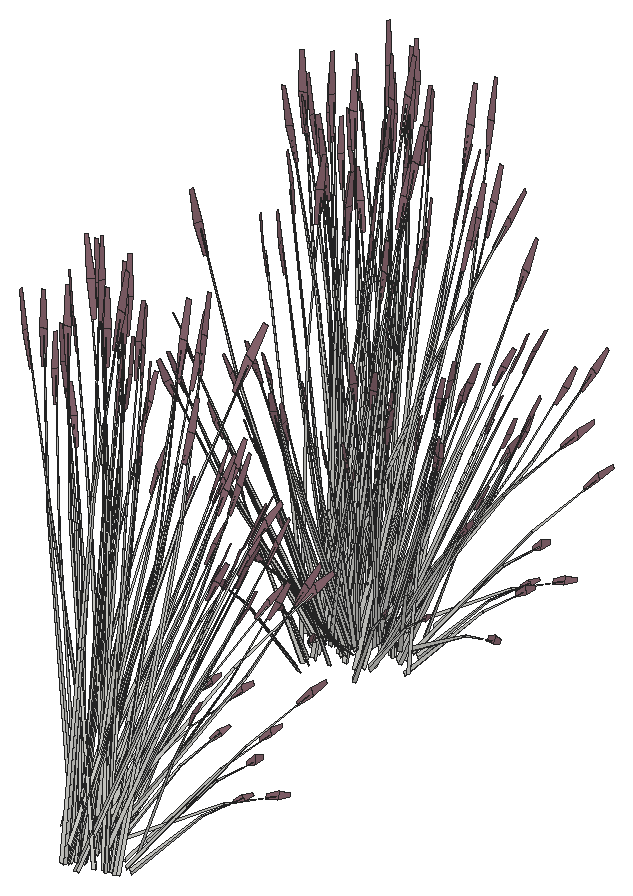
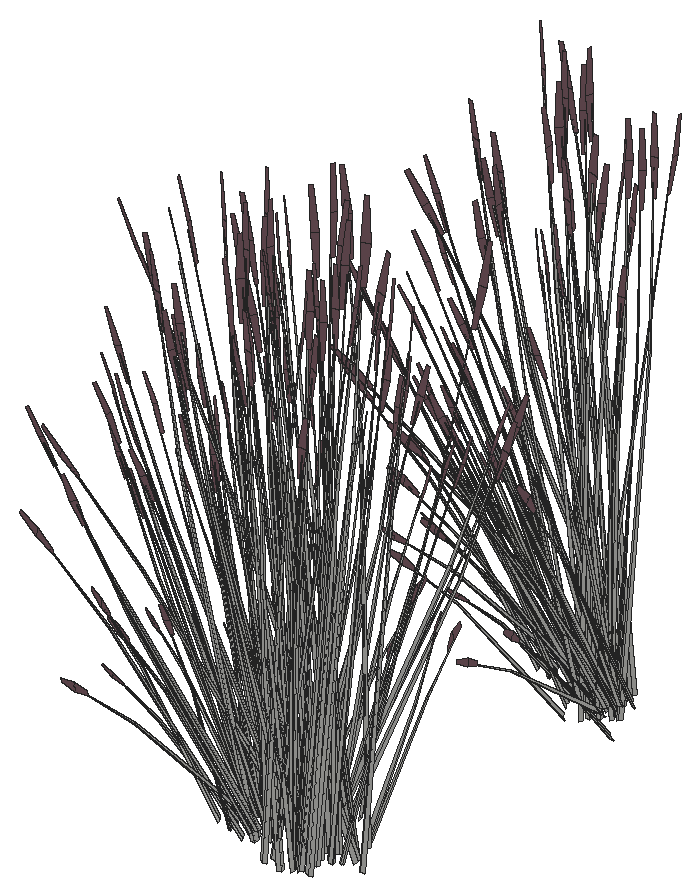
# SketchUp Ruby script. Lengths in inches.
U = 1.inch
M = Sketchup.active_model
def pt(a) = Geom::Point3d.new(a.map { |v| v * U })
def face(e, loops, mat)
  f = e.add_face(loops[0].map { |a| pt(a) })
  loops[1..].each { |l| e.add_face(l.map { |a| pt(a) }).erase! }
  f.material = f.back_material = mat if mat
  f
end
# faces: each face lists its corners as indices into pts; further lists are holes
def faces(e, pts, list, mat = nil) = list.each { |f| face(e, (f[0].is_a?(Array) ? f : [f]).map { |l| l.map { |i| pts[i] } }, mat) }
# xy, xz, yz: faces in a plane at the given z, y or x. An outline is a flat list of corners, or four numbers for a rectangle; further outlines are holes
def ring(l) = l.size == 4 ? [[l[0], l[1]], [l[2], l[1]], [l[2], l[3]], [l[0], l[3]]] : l.each_slice(2).to_a
def flat(e, list, mat, &to3) = list.each { |f| face(e, (f[0].is_a?(Array) ? f : [f]).map { |l| ring(l).map { |u, v| to3.(u, v) } }, mat) }
def xy(e, z, list, mat = nil) = flat(e, list, mat) { |x, y| [x, y, z] }
def xz(e, y, list, mat = nil) = flat(e, list, mat) { |x, z| [x, y, z] }
def yz(e, x, list, mat = nil) = flat(e, list, mat) { |y, z| [x, y, z] }
def lines(e, pts, list) = list.each { |a, b| e.add_line(pt(pts[a]), pt(pts[b])) }
# prism: a flat outline (further loops are holes) pulled along v
def prism(e, loops, v, mat = nil)
  f = face(e, loops, mat); d = Geom::Vector3d.new(v.map { |x| x * U })
  f.pushpull(f.normal.samedirection?(d) ? d.length : -d.length)
end
def box(e, o, s, mat = nil) = prism(e, [[o, [o[0] + s[0], o[1], o[2]], [o[0] + s[0], o[1] + s[1], o[2]], [o[0], o[1] + s[1], o[2]]]], [0, 0, s[2]], mat)
def at(x, y, z, deg = 0) = Geom::Transformation.translation(pt([x, y, z])) * Geom::Transformation.rotation(ORIGIN, Z_AXIS, deg.degrees)
def axes(o, x, y, z) = Geom::Transformation.new([*x, 0, *y, 0, *z, 0, *pt(o).to_a, 1])
def part(name) = M.definitions.add(name)
# library, detail: a bought-in or finely detailed component or shape, given as its bounding box
def library(name, o, s) = part(name).tap { |d| box(d.entities, o, s) }
def detail(e, o, s) = box(e.add_group.entities, o, s)
def put(e, d, t, mat = nil) = e.add_instance(d, t).tap { |i| i.material = mat if mat }
def group(e, t, mat = nil) = e.add_group.tap { |g| g.transformation = t; g.material = mat if mat }.entities
root = M.entities
M.materials.add("LightPink_Translucent").color = [144, 107, 117]
c1 = part("blade")
p = [[2.15,0.21,22],[0,0.17,0],[0.09,0.45,0],[2.18,0.31,22],[2.29,0.31,22],[0.38,0.45,0],
  [2.48,0.24,33],[2.49,0.24,33],[2.48,0.22,33]]
faces(c1.entities,p,[[0,1,2,3],[4,5,2,3],[6,3,4,7],[8,0,3,6]])
c2 = part("seeds")
p = [[0.3,-0.1,1.38],[-0.01,-0.03,1.59],[-0.01,-0.03,0.03],[0.14,-0.07,-0.07],[0.29,-0.03,3],[0.15,0.01,3.11]]
faces(c2.entities,p,[[0,1,2,3],[1,0,4,5]],"LightPink_Translucent")
c3 = part("blade with seeds")
put(c3.entities,c1,at(0,0,0))
put(c3.entities,c2,axes([2.4,0.25,30.99],[1.5799,-0.05474,1.17369],[-0.12525,1.92788,0.29478],[-0.07173,-0.02425,1.56792]))
put(root,c3,axes([73.33,431.42,34.53],[-0.50328,-1.06202,-0.69835],[1.44974,-0.38248,-0.18329],[-0.05563,-0.35963,1.54149]))
put(root,c3,axes([76.63,428.04,37.46],[-1.19922,0.48218,-0.1216],[-0.58932,-0.85579,-0.67495],[-0.15822,-0.36063,1.02557]))
put(root,c3,axes([75.6,428.08,37.11],[-1.20468,-0.25962,-0.51099],[0.41292,-0.89013,-0.3958],[-0.11046,-0.35838,0.97773]))
put(root,c3,axes([73.38,392.2,32.11],[-0.02999,-0.3975,1.71376],[1.30002,0.26369,0.13857],[-0.08041,0.56647,0.73262]))
put(root,c3,axes([70.95,431.29,34.46],[0.85545,-0.64616,-0.30978],[0.85545,0.64616,0.30978],[0,-0.20813,1.38974]))
put(root,c3,axes([74.82,427.11,34.56],[-0.84686,0.59414,-0.03893],[-0.77596,-0.65071,-0.17649],[-0.05463,-0.18438,0.58215]))
put(root,c3,axes([74.48,432.97,34.79],[1.54892,0.2182,0.45755],[-0.31522,1.23236,0.17955],[-0.22636,-0.119,1.58856]))
put(root,c3,axes([74.08,432.75,35.15],[-0.59459,0.93321,0.44739],[-1.23546,-0.44912,-0.21531],[0,-0.21512,1.43643]))
put(root,c3,axes([76.04,428.25,37.41],[-0.5849,-0.8421,-0.71045],[1.20401,-0.4693,0.08574],[-0.13677,-0.40688,1.00501]))
put(root,c3,axes([73.65,434.94,34.9],[1.31687,-0.27488,0.17642],[0.32517,1.02297,0.35086],[-0.11745,-0.14905,1.60407]))
put(root,c3,axes([75.34,392.62,30.43],[-1.23546,-0.46496,0],[0.59459,-0.96613,0],[0,0,1.62707]))
put(root,c3,axes([75.34,435.1,34.625],[-1.23546,-0.46496,0],[0.59459,-0.96613,0],[0,0,1.62707]))
put(root,c3,axes([76.27,428.375,37.48],[-0.36946,0.79643,0.35414],[-1.07787,-0.23229,-0.4572],[-0.09883,-0.32066,0.87481]))
put(root,c3,axes([78.2,393.78,30.61],[0.7662,1.03778,0],[-1.28187,0.57875,-0.51607],[-0.29196,0.13181,1.63711]))
put(root,c3,axes([74.3,394.23,33.3],[-1.20755,-0.27075,0.53283],[0.41292,-0.89013,0.43934],[0.07257,0.35005,1.10256]))
put(root,c3,axes([73.98,394.3,32.97],[-0.90301,0.35198,0.0643],[-0.44199,-0.64184,0.50621],[0.08721,0.28293,0.77189]))
put(root,c3,axes([77.5625,392.51,30.71],[0.35402,-1.02926,0.17642],[1.29548,0.29127,0.35086],[-0.22379,0.00501,1.60407]))
put(root,c3,axes([77.5625,435,34.9],[0.35402,-1.02926,0.17642],[1.29548,0.29127,0.35086],[-0.22379,0.00501,1.60407]))
put(root,c3,axes([76.97,391.15,30.85],[0.90538,0.62224,0.1448],[-0.75521,0.70202,-0.41347],[-0.21021,0.09491,1.26744]))
put(root,c3,axes([76.97,433.63,35.04],[0.90538,0.62224,0.1448],[-0.75521,0.70202,-0.41347],[-0.21021,0.09491,1.26744]))
put(root,c3,axes([76.64,432.86,34.73],[-1.1399,-0.8914,-0.06131],[1.1406,-0.89194,0],[-0.03981,-0.03113,1.75571]))
put(root,c3,axes([76.94,390.6875,30.95],[1.33077,-0.06393,0.44739],[0.12035,1.06125,-0.21531],[-0.23824,0.10756,1.43643]))
put(root,c3,axes([76.94,433.17,35.15],[1.33077,-0.06393,0.44739],[0.12035,1.06125,-0.21531],[-0.23824,0.10756,1.43643]))
put(root,c3,axes([77.27,393.13,30.57],[1.53422,0.33662,0.30756],[-0.38383,1.20322,-0.36492],[-0.25393,0.15059,1.64885]))
put(root,c3,axes([75.03,426.38,33.92],[-0.20555,0.03731,1.76342],[-1.13672,-0.42002,-0.26939],[0.01907,-0.35034,0.30037]))
put(root,c3,axes([77.93,393.0625,30.71],[1.14694,-0.51783,0.49651],[0.68554,0.92854,0],[-0.26122,0.11794,1.57504]))
put(root,c3,axes([77.93,435.55,34.91],[1.14694,-0.51783,0.49651],[0.68554,0.92854,0],[-0.26122,0.11794,1.57504]))
put(root,c3,axes([76.15,427.54,36.95],[0.36946,-0.79643,-0.35414],[1.07787,0.23229,0.4572],[-0.09883,-0.32066,0.87481]))
put(root,c3,axes([74.34,431.84,34.79],[0.53281,1.15808,0.45755],[-1.52239,0.4027,0.17955],[0.01861,-0.2128,1.58856]))
put(root,c3,axes([74.1,431.6875,34.64],[0.59459,-0.93321,-0.44739],[1.23546,0.44912,0.21531],[0,-0.21512,1.43643]))
put(root,c3,axes([75.62,392.21,30.44],[-0.39985,-0.89288,0],[1.1418,-0.31268,0],[0,0,1.54371]))
put(root,c3,axes([75.62,434.7,34.63],[-0.39985,-0.89288,0],[1.1418,-0.31268,0],[0,0,1.54371]))
put(root,c3,axes([74.17,394.1,29.73],[0.19833,-0.05635,1.76342],[1.19302,0.31018,-0.26939],[0.03489,0.3496,0.30037]))
put(root,c3,axes([74.43,394.41,32.76],[-0.36946,0.79643,-0.35414],[-1.07787,-0.23229,0.4572],[0.09883,0.32066,0.87481]))
put(root,c3,axes([77.24,390.45,30.45],[-0.59459,0.93321,-0.44739],[-1.23546,-0.44912,0.21531],[0,0.21512,1.43643]))
put(root,c3,axes([76.6,427.65,37.16],[0.90301,-0.35198,0.0643],[0.44199,0.64184,0.50621],[-0.08721,-0.28293,0.77189]))
put(root,c3,axes([73.67,395.82,32.95],[0.15534,0.16677,1.74944],[1.25362,0.06552,-0.27667],[0.12606,0.3678,0.14031]))
put(root,c3,axes([79.59,389.89,30.71],[-0.96285,-0.75439,0.17642],[0.97031,-0.7317,0.35086],[-0.10634,0.15406,1.60407]))
put(root,c3,axes([79.59,432.37,34.9],[-0.96285,-0.75439,0.17642],[0.97031,-0.7317,0.35086],[-0.10634,0.15406,1.60407]))
put(root,c3,axes([76.26,431.93,34.63],[0,-1.19833,0],[1.53239,0,0],[0,0,1.79456]))
put(root,c3,axes([76.28,427.72,37.16],[1.20755,0.27075,0.48003],[-0.41292,0.89013,0.3958],[-0.07257,-0.35005,0.9933]))
put(root,c3,axes([74.84,432.15,34.86],[1.3808,0.50196,0.24065],[-0.66454,1.04299,0.50002],[0,-0.24043,1.60543]))
put(root,c3,axes([77.03,389.93,30.53],[0,1.19774,-0.05637],[-1.53239,0,0],[0,0.03764,1.79368]))
put(root,c3,axes([77.03,432.41,34.72],[0,1.19774,-0.05637],[-1.53239,0,0],[0,0.03764,1.79368]))
put(root,c3,axes([74.39,431.45,35.15],[-1.33077,0.06393,0.44739],[-0.12035,-1.06125,-0.21531],[0.23824,-0.10756,1.43643]))
put(root,c3,axes([74.3125,393.57,33.29],[0.36946,-0.79643,0.35414],[1.07787,0.23229,-0.4572],[0.09883,0.32066,0.87481]))
put(root,c3,axes([73.77,429.63,34.9],[-0.35402,1.02926,0.17642],[-1.29548,-0.29127,0.35086],[0.22379,-0.00501,1.60407]))
put(root,c3,axes([76.3,392.25,30.53],[0.53281,1.18979,-0.06012],[-1.52239,0.41691,0],[0.01861,0.04155,1.72173]))
put(root,c3,axes([76.3,434.73,34.72],[0.53281,1.18979,-0.06012],[-1.52239,0.41691,0],[0.01861,0.04155,1.72173]))
put(root,c3,axes([73.14,428.36,34.8],[-0.7662,-1.03778,0],[1.28187,-0.57875,-0.51607],[0.29196,-0.13181,1.63711]))
put(root,c3,axes([74.54,393.7,33.22],[0.5849,0.8421,-0.71045],[-1.20401,0.4693,0.08574],[0.13677,0.40688,1.00501]))
put(root,c3,axes([80.7,390.69,30.4375],[-1.53164,-0.00828,-0.04976],[0,-1.1575,0.49943],[-0.04813,0.2635,1.58352]))
put(root,c3,axes([80.7,433.17,34.63],[-1.53164,-0.00828,-0.04976],[0,-1.1575,0.49943],[-0.04813,0.2635,1.58352]))
put(root,c3,axes([77.6875,429.6875,34.9],[-1.31687,0.27488,0.17642],[-0.32517,-1.02297,0.35086],[0.11745,0.14905,1.60407]))
put(root,c3,axes([76.34,425.85,35.19],[0.15721,0.60392,1.1486],[-0.87211,-0.33448,0.84392],[0.09385,-0.30923,0.25299]))
put(root,c3,axes([75.76,396.42,33.88],[0.84686,-0.59414,-0.06488],[0.77596,0.65071,-0.29416],[0.05463,0.18438,0.97024]))
put(root,c3,axes([75.53,431.18,34.79],[-1.01611,0.93987,0.45755],[-1.20717,-0.82966,0.17955],[0.24496,-0.0938,1.58856]))
put(root,c3,axes([77.27,390.18,30.45],[0.85545,0.66896,0],[-0.85545,0.66896,0],[0,0,1.69266]))
put(root,c3,axes([77.27,432.66,34.64],[0.85545,0.66896,0],[-0.85545,0.66896,0],[0,0,1.69266]))
put(root,c3,axes([77.26,389.39,30.95],[0.59459,-0.93321,0.44739],[1.23546,0.44912,-0.21531],[0,0.21512,1.43643]))
put(root,c3,axes([77.26,431.88,35.15],[0.59459,-0.93321,0.44739],[1.23546,0.44912,-0.21531],[0,0.21512,1.43643]))
put(root,c3,axes([76.74,392.64,30.44],[1.23546,0.46496,0],[-0.59459,0.96613,0],[0,0,1.74954]))
put(root,c3,axes([76.74,435.12,34.63],[1.23546,0.46496,0],[-0.59459,0.96613,0],[0,0,1.74954]))
put(root,c3,axes([74.98,393.87,32.92],[1.20468,0.25962,-0.51099],[-0.41292,0.89013,-0.3958],[0.11046,0.35838,0.97773]))
put(root,c3,axes([73.95,393.91,33.27],[1.19922,-0.48218,-0.1216],[0.58932,0.85579,-0.67495],[0.15822,0.36063,1.02557]))
put(root,c3,axes([76.86,389.17,30.62],[-1.54892,-0.2182,0.49198],[0.31522,-1.23236,0.19306],[0.22636,0.119,1.70813]))
put(root,c3,axes([76.86,431.66,34.81],[-1.54892,-0.2182,0.49198],[0.31522,-1.23236,0.19306],[0.22636,0.119,1.70813]))
put(root,c3,axes([80.08,426.84,37.14],[-0.12446,0.07911,1.77383],[-1.21937,-0.26689,-0.16761],[-0.04414,-0.34521,0.31391]))
put(root,c3,axes([79.12,429.125,37.46],[-1.34686,-0.05131,-0.1216],[0.03681,-0.97156,-0.67495],[0.09356,-0.37418,1.02557]))
put(root,c3,axes([80.38,390.85,30.26],[-0.85545,0.64616,-0.30978],[-0.85545,-0.64616,0.30978],[0,0.20813,1.38974]))
put(root,c3,axes([77.94,390.73,30.33],[0.44936,0.94823,-0.69212],[-1.29441,0.3415,-0.18165],[0.04967,0.32109,1.52773]))
put(root,c3,axes([77.3,432.2,34.63],[1.37109,0,0],[0,1.07219,0],[0,0,1.78407]))
put(root,c3,axes([78.59,429.27,37.48],[-0.82919,0.54528,0.35414],[-0.78493,-0.62262,-0.4572],[0.11943,-0.31634,0.87481]))
put(root,c3,axes([75.98,431.02,35.15],[-0.73619,-0.86927,0.44739],[1.11511,-0.61213,-0.21531],[0.23824,0.10756,1.43643]))
put(root,c3,axes([74.64,431.23,35.09],[-0.1428,-1.18174,-0.29095],[1.48733,-0.07145,-0.50002],[0.26191,-0.15741,1.59708]))
put(root,c3,axes([77.77,389.61,30.85],[1.1418,-0.30203,0.1448],[0.39985,0.86246,-0.41347],[0,0.18981,1.26744]))
put(root,c3,axes([77.77,432.09,35.04],[1.1418,-0.30203,0.1448],[0.39985,0.86246,-0.41347],[0,0.18981,1.26744]))
put(root,c3,axes([78.2,428.76,37.11],[-0.87728,-0.69587,-0.51099],[0.92674,-0.60943,-0.3958],[0.13348,-0.35356,0.97773]))
put(root,c3,axes([77.38,389.68,30.9],[1.38012,0.49416,-0.29095],[-0.66454,1.04299,-0.50002],[0.04337,0.25608,1.59708]))
put(root,c3,axes([77.38,432.16,35.09],[1.38012,0.49416,-0.29095],[-0.66454,1.04299,-0.50002],[0.04337,0.25608,1.59708]))
put(root,c3,axes([74.45,428.61,34.46],[1.14332,0.25625,-0.30978],[-0.28787,0.90242,0.30978],[0.23049,-0.10406,1.38974]))
put(root,c3,axes([77.625,427.52,35.02],[-0.34835,0.20963,1.43002],[-1.04325,-0.36691,-0.30754],[0.19338,-0.4563,0.61141]))
put(root,c3,axes([80.38,389.91,30.71],[0,-1.03566,0.49651],[1.37109,0,0],[0,0.23588,1.57504]))
put(root,c3,axes([80.38,432.4,34.91],[0,-1.03566,0.49651],[1.37109,0,0],[0,0.23588,1.57504]))
put(root,c3,axes([80.97,390.875,30.25],[0,1.03566,-0.49651],[-1.37109,0,0],[0,0.23588,1.57504]))
put(root,c3,axes([77.31,394.01,32.97],[-1.21888,0.23767,0.48003],[-0.21154,-0.93233,0.3958],[0.28666,0.27478,0.9933]))
put(root,c3,axes([74.18,428.2,34.45],[1.14694,-0.51783,-0.49651],[0.68554,0.92854,0],[0.26122,-0.11794,1.57504]))
put(root,c3,axes([77.07,394.2,32.97],[-0.55698,0.6579,0.0643],[-0.79316,-0.38303,0.50621],[0.25643,0.21093,0.77189]))
put(root,c3,axes([75.66,392.03,32.11],[-0.28013,-0.33252,1.71376],[1.29445,-0.27994,0.13857],[0.29256,0.52202,0.73262]))
put(root,c3,axes([76.48,430.78,35.04],[0.23642,-0.92427,0.1448],[1.15506,0.16044,-0.41347],[0.21021,0.09491,1.26744]))
put(root,c3,axes([78.12,429.17,34.91],[-1.14694,-0.51783,0.49651],[0.68554,-0.92854,0],[0.26122,0.11794,1.57504]))
put(root,c3,axes([78.47,429.08,37.41],[0.03189,-0.95798,-0.71045],[1.34277,0.06434,0.08574],[0.14171,-0.40585,1.00501]))
put(root,c3,axes([77.12,392.09,30.42],[1.2866,-0.3514,-0.19198],[0.45209,1.01223,0.00008],[0.14202,-0.03884,1.73897]))
put(root,c3,axes([77.12,434.57,34.61],[1.2866,-0.3514,-0.19198],[0.45209,1.01223,0.00008],[0.14202,-0.03884,1.73897]))
put(root,c3,axes([76.9,393.44,33.29],[-0.18927,-0.83419,0.35414],[1.08199,-0.22027,-0.4572],[0.29062,0.23905,0.87481]))
put(root,c3,axes([77.14,389.08,30.45],[0.73619,0.86927,-0.44739],[-1.11511,0.61213,0.21531],[0.23824,0.10756,1.43643]))
put(root,c3,axes([77.14,431.5625,34.64],[0.73619,0.86927,-0.44739],[-1.11511,0.61213,0.21531],[0.23824,0.10756,1.43643]))
put(root,c3,axes([77.63,388.64,32.71],[-1.05895,-0.53811,1.38283],[1.11816,-0.83781,0.59665],[0.34166,0.5049,1.33663]))
put(root,c3,axes([79.03,428.5,36.95],[0.82919,-0.54528,-0.35414],[0.78493,0.62262,0.4572],[0.11943,-0.31634,0.87481]))
put(root,c3,axes([75.85,394.61,32.95],[0.00363,-0.12539,1.77383],[1.0502,-0.55319,-0.16761],[0.36479,0.19745,0.31391]))
put(root,c3,axes([79.35,428.78,37.16],[1.00708,0.04826,0.0643],[-0.02761,0.72867,0.50621],[0.10538,-0.27912,0.77189]))
put(root,c3,axes([79.23,393.02,31],[-0.69001,-0.29779,1.1486],[0.89096,-0.30257,0.84392],[0.24031,0.2563,0.25299]))
put(root,c3,axes([76.77,392.71,30.83],[0.02163,-0.34331,1.43002],[1.03345,-0.38348,-0.30754],[0.31903,0.4109,0.61141]))
put(root,c3,axes([80.35,427.58,37.14],[-0.01183,-0.20612,1.74944],[-0.99913,-0.59572,-0.27667],[0.15447,-0.36112,0.14031]))
put(root,c3,axes([75.54,430.32,34.49],[0.82544,-0.77843,-0.62353],[1.0254,0.70586,-0.16365],[0.33076,-0.19418,1.37633]))
put(root,c3,axes([79.02,428.71,37.16],[0.87265,0.70663,0.48003],[-0.92674,0.60943,0.3958],[0.16097,-0.33153,0.9933]))
put(root,c3,axes([79.16,429.63,34.46],[0.28787,0.90242,-0.30978],[-1.14332,0.25625,0.30978],[0.23049,0.10406,1.38974]))
put(root,c3,axes([81.31,390.09,30.61],[1.53239,0,0],[0,1.1575,-0.51607],[0,0.26363,1.63711]))
put(root,c3,axes([81.31,432.58,34.8],[1.53239,0,0],[0,1.1575,-0.51607],[0,0.26363,1.63711]))
put(root,c3,axes([76.36,431.08,35.09],[1.23732,-0.68758,-0.29095],[0.8228,0.97154,-0.50002],[0.30528,0.09867,1.59708]))
put(root,c3,axes([79.34,394.38,30.9],[-0.78586,-0.03248,1.0506],[0.51898,-0.68985,0.58006],[0.31045,0.24509,0.8241]))
put(root,c3,axes([80.03,430.96,37.48],[-1.06674,0.14801,0.35414],[-0.28168,-0.84611,-0.4572],[0.30569,-0.22726,0.87481]))
put(root,c3,axes([76.96,428.59,36.3],[-0.22818,0.35597,1.71376],[-0.95725,-0.73667,0.13857],[0.43183,-0.45914,0.73262]))
put(root,c3,axes([76.8,393.875,33.27],[0.73026,-0.88648,-0.1216],[1.05755,0.51071,-0.67495],[0.36761,0.25045,1.02557]))
put(root,c3,axes([73.23,430.46,34.02],[-1.20625,0.41464,1.28929],[-0.38394,-1.1897,0.50096],[0.74071,0.01979,1.46642]))
put(root,c3,axes([80.59,431.04,37.46],[-1.1336,-0.57106,-0.1216],[0.65308,-0.827,-0.67495],[0.32027,-0.28747,1.02557]))
put(root,c3,axes([77.67,393.43,32.92],[1.20928,-0.24619,-0.51099],[0.21154,0.93233,-0.3958],[0.32481,0.26718,0.97773]))
put(root,c3,axes([78.78,428.625,34.8],[0.7662,-1.03778,0],[1.28187,0.57875,-0.51607],[0.29196,0.13181,1.63711]))
put(root,c3,axes([80.0625,428.17,33.92],[-0.18342,-0.08159,1.76342],[-0.47115,-0.9115,-0.26939],[0.31784,-0.24736,0.30037]))
put(root,c3,axes([79.06,392.32,33.29],[-0.69728,-0.64842,0.35414],[0.79619,-0.61382,-0.4572],[0.40453,0.09339,0.87481]))
put(root,c3,axes([79.06,434.8,37.48],[-0.69728,-0.64842,0.35414],[0.79619,-0.61382,-0.4572],[0.40453,0.09339,0.87481]))
put(root,c3,axes([79.48,429.25,34.45],[1.14694,0.51783,-0.49651],[-0.68554,0.92854,0],[0.26122,0.11794,1.57504]))
put(root,c3,axes([79.6875,392.9,32.97],[-0.06171,0.78753,0.0643],[-0.9318,-0.02159,0.50621],[0.35694,0.08241,0.77189]))
put(root,c3,axes([79.42,394.13,29.73],[0.08928,-0.14952,1.76342],[1.12407,-0.44035,-0.26939],[0.34078,0.22791,0.30037]))
put(root,c3,axes([79.77,392.65,32.97],[-0.90362,0.68241,0.48003],[-0.77932,-0.72471,0.3958],[0.42395,0.12588,0.9933]))
put(root,c3,axes([80.02,430.36,37.11],[-0.31482,-0.94565,-0.51099],[1.19224,-0.16542,-0.3958],[0.34166,-0.254,0.97773]))
put(root,c3,axes([82.12,392.75,32.17],[-0.23455,-0.87059,-0.03492],[1.10861,-0.20015,-0.15832],[0.23151,0.05519,0.52218]))
put(root,c3,axes([82.12,435.24,36.36],[-0.23455,-0.87059,-0.03492],[1.10861,-0.20015,-0.15832],[0.23151,0.05519,0.52218]))
put(root,c3,axes([80.2,432.98,37.48],[-1.01846,-0.28891,0.35414],[0.29705,-0.84289,-0.4572],[0.41005,-0.07729,0.87481]))
put(root,c3,axes([77.8,388.75,30.3],[1.27479,0.1698,-0.62353],[-0.26901,1.04736,-0.16365],[0.38043,0.12691,1.37633]))
put(root,c3,axes([77.8,431.23,34.49],[1.27479,0.1698,-0.62353],[-0.26901,1.04736,-0.16365],[0.38043,0.12691,1.37633]))
put(root,c3,axes([83.23,431.85,34.6875],[-0.75977,-0.66224,-0.06488],[0.83212,-0.6068,-0.29416],[0.23578,-0.04272,0.97024]))
put(root,c3,axes([81.49,428.48,35.19],[-0.40819,0.5272,1.1486],[-0.35086,-0.70831,0.84392],[0.33713,-0.17749,0.25299]))
put(root,c3,axes([81,430.82,37.16],[0.8413,0.43556,0.0643],[-0.48981,0.62025,0.50621],[0.26973,-0.20053,0.77189]))
put(root,c3,axes([80.77,430.64,37.16],[0.30393,0.95317,0.48003],[-1.19224,0.16542,0.3958],[0.35138,-0.22417,0.9933]))
put(root,c3,axes([77.54,390.99,32.11],[-0.45521,-0.17844,1.71376],[0.94204,-0.74856,0.13857],[0.58713,0.33769,0.73262]))
put(root,c3,axes([83.38,430.79,37.14],[-0.16006,-0.00787,1.77383],[-0.66468,-0.8428,-0.16761],[0.26693,-0.27711,0.31391]))
put(root,c3,axes([80.9,430.46,36.95],[1.06674,-0.14801,-0.35414],[0.28168,0.84611,0.4572],[0.30569,-0.22726,0.87481]))
put(root,c3,axes([80.06,430.74,37.41],[0.64013,-0.81717,-0.71045],[1.12174,0.58074,0.08574],[0.38221,-0.29607,1.00501]))
put(root,c3,axes([81.125,433.24,37.16],[0.4501,0.70615,0.0643],[-0.82077,0.34564,0.50621],[0.36181,-0.0682,0.77189]))
put(root,c3,axes([80.05,392.65,32.76],[0.69728,0.64842,-0.35414],[-0.79619,0.61382,0.4572],[0.40453,0.09339,0.87481]))
put(root,c3,axes([80.05,435.14,36.95],[0.69728,0.64842,-0.35414],[-0.79619,0.61382,0.4572],[0.40453,0.09339,0.87481]))
put(root,c3,axes([79.25,392.73,33.27],[0.06562,-1.05324,-0.1216],[1.2424,0.02879,-0.67495],[0.4785,0.07316,1.02557]))
put(root,c3,axes([79.25,435.21,37.46],[0.06562,-1.05324,-0.1216],[1.2424,0.02879,-0.67495],[0.4785,0.07316,1.02557]))
put(root,c3,axes([80.63,433.26,37.46],[-0.6166,-0.93779,-0.1216],[1.09436,-0.46085,-0.67495],[0.46117,-0.12373,1.02557]))
put(root,c3,axes([81.04,390.51,32.97],[-0.34623,0.9443,0.48003],[-1.13828,-0.3229,0.3958],[0.44763,-0.05675,0.9933]))
put(root,c3,axes([81.04,432.99,37.16],[-0.34623,0.9443,0.48003],[-1.13828,-0.3229,0.3958],[0.44763,-0.05675,0.9933]))
put(root,c3,axes([80.33,392.1,32.95],[0.26289,-0.01751,1.74944],[0.72108,-0.8046,-0.27667],[0.46761,0.10621,0.14031]))
put(root,c3,axes([80.33,434.58,37.14],[0.26289,-0.01751,1.74944],[0.72108,-0.8046,-0.27667],[0.46761,0.10621,0.14031]))
put(root,c3,axes([80.58,432.46,37.11],[0.332,-0.94205,-0.51099],[1.13828,0.3229,-0.3958],[0.45829,-0.08638,0.97773]))
put(root,c3,axes([83.4375,390.58,31],[-0.75718,0.17097,1.1486],[0.35641,-0.70661,0.84392],[0.40168,0.04835,0.25299]))
put(root,c3,axes([83.4375,433.06,35.19],[-0.75718,0.17097,1.1486],[0.35641,-0.70661,0.84392],[0.40168,0.04835,0.25299]))
put(root,c3,axes([80.98,429.99,35.02],[-0.4378,-0.03068,1.43002],[-0.44851,-0.8229,-0.30754],[0.53783,-0.23279,0.61141]))
put(root,c3,axes([81.28,432.89,36.95],[1.01846,0.28891,-0.35414],[-0.29705,0.84289,0.4572],[0.41005,-0.07729,0.87481]))
put(root,c3,axes([79.31,392.22,33.22],[1.22504,0.02494,-0.71045],[-0.08228,1.05005,0.08574],[0.51899,0.11081,1.00501]))
put(root,c3,axes([79.31,434.71,37.41],[1.22504,0.02494,-0.71045],[-0.08228,1.05005,0.08574],[0.51899,0.11081,1.00501]))
put(root,c3,axes([81.79,432.72,34.41],[-0.7893,0.12429,1.41583],[-0.12563,-0.9893,0.08104],[0.55282,-0.14974,0.80566]))
put(root,c3,axes([82.66,432.08,33.92],[-0.06405,-0.15723,1.76342],[0.44421,-0.91974,-0.26939],[0.4481,-0.01323,0.30037]))
put(root,c3,axes([83.08,393.57,32.95],[-0.11081,-0.09067,1.77383],[0.2424,-0.97188,-0.16761],[0.43649,-0.06209,0.31391]))
put(root,c3,axes([83.08,436.05,37.14],[-0.11081,-0.09067,1.77383],[0.2424,-0.97188,-0.16761],[0.43649,-0.06209,0.31391]))
put(root,c3,axes([78.5,431.85,36.3],[-0.50831,0.02346,1.71376],[0.33721,-1.01661,0.13857],[0.72439,0.06288,0.73262]))
put(root,c3,axes([80.36,432.8,37.41],[1.07686,-0.45739,-0.71045],[0.60013,0.94154,0.08574],[0.52031,-0.10696,1.00501]))
put(root,c3,axes([83.98,431.79,37.14],[0.17006,-0.15775,1.74944],[-0.21766,-0.96766,-0.27667],[0.42669,-0.18347,0.14031]))
put(root,c3,axes([82.02,391.71,30.83],[-0.29514,-0.25472,1.43002],[0.38401,-0.84262,-0.30754],[0.59714,0.11414,0.61141]))
put(root,c3,axes([82.02,434.19,35.02],[-0.29514,-0.25472,1.43002],[0.38401,-0.84262,-0.30754],[0.59714,0.11414,0.61141]))
